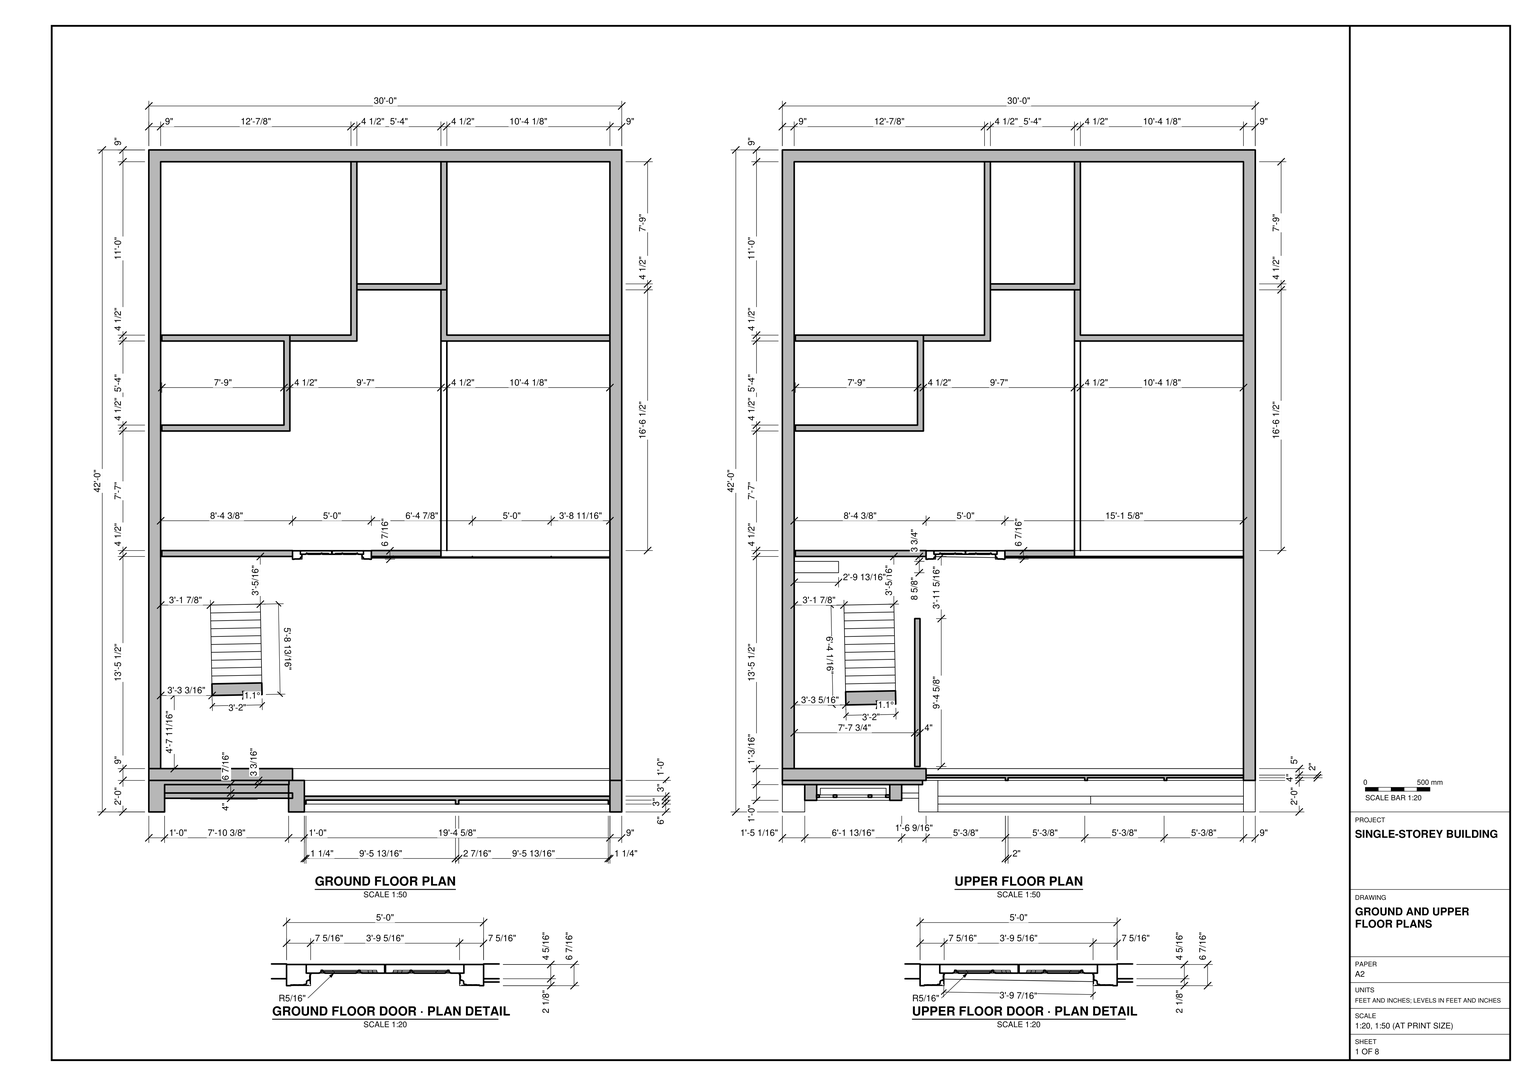
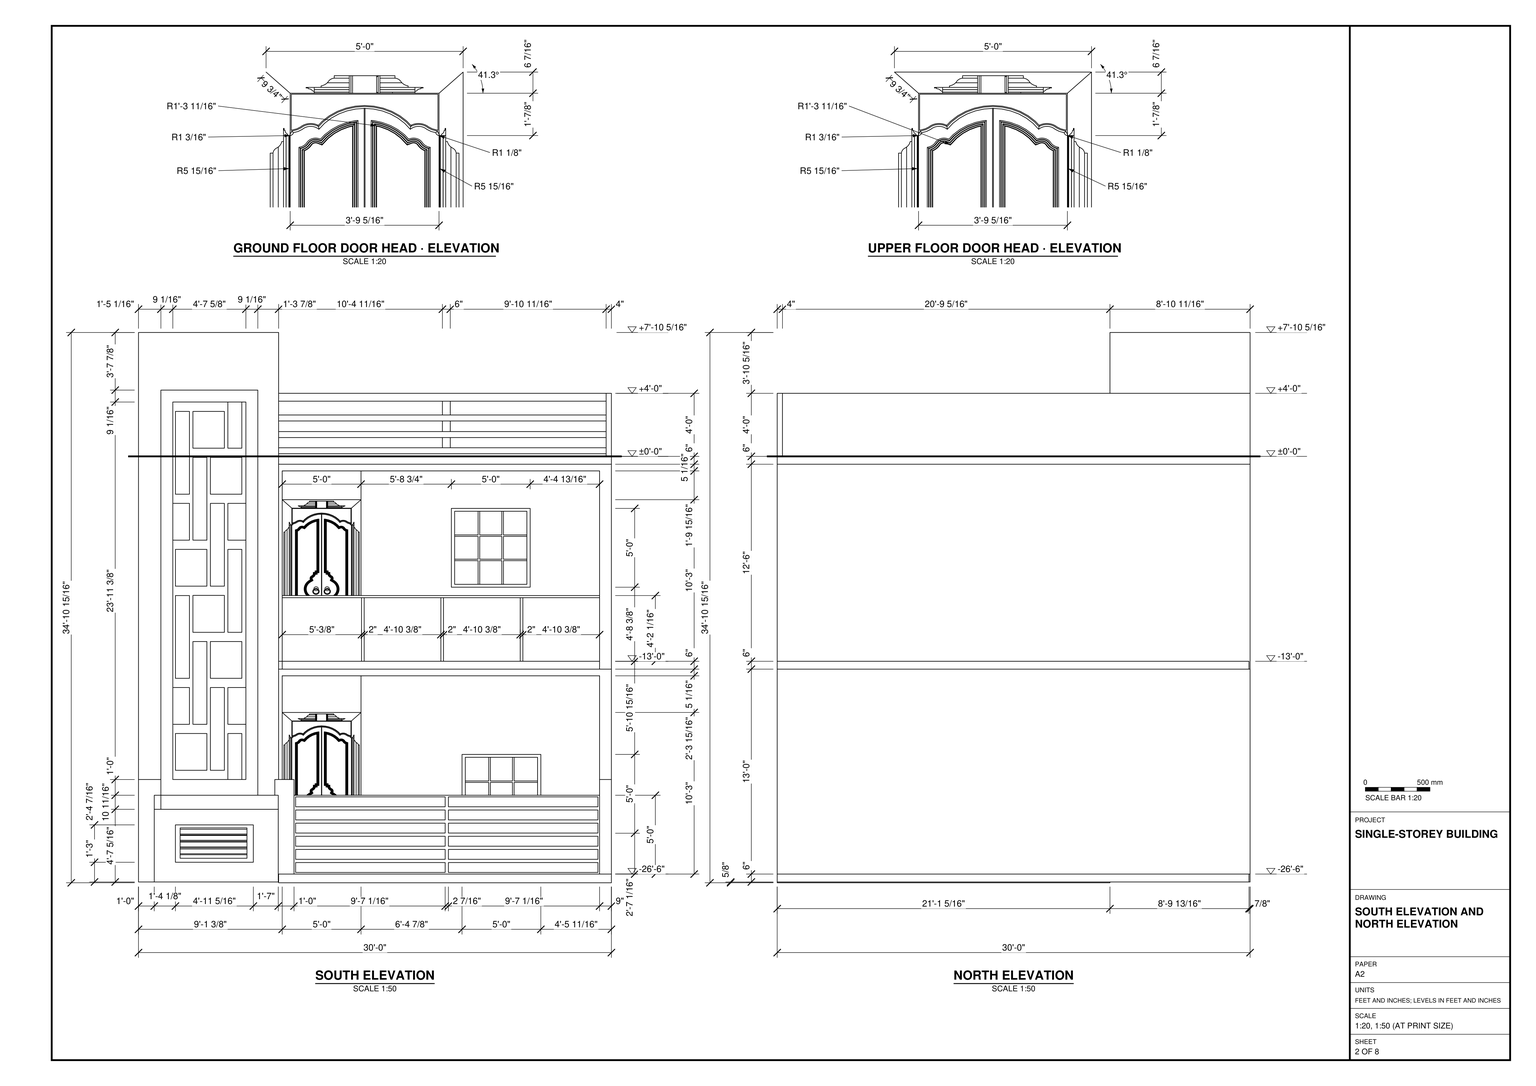
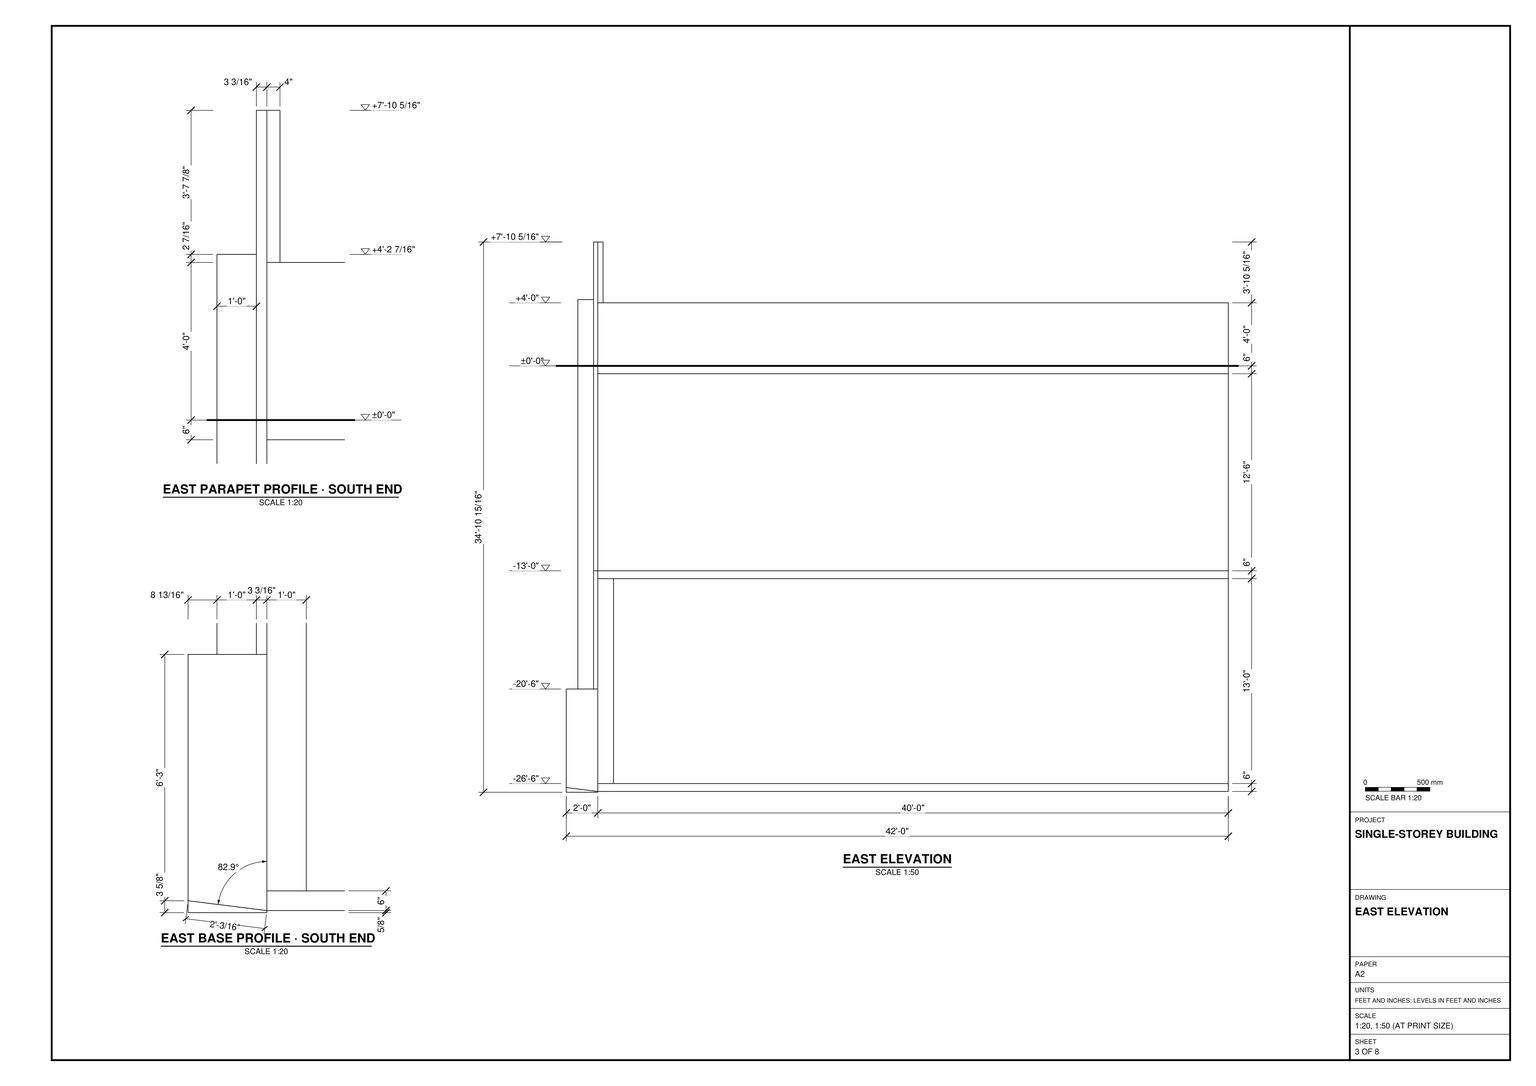
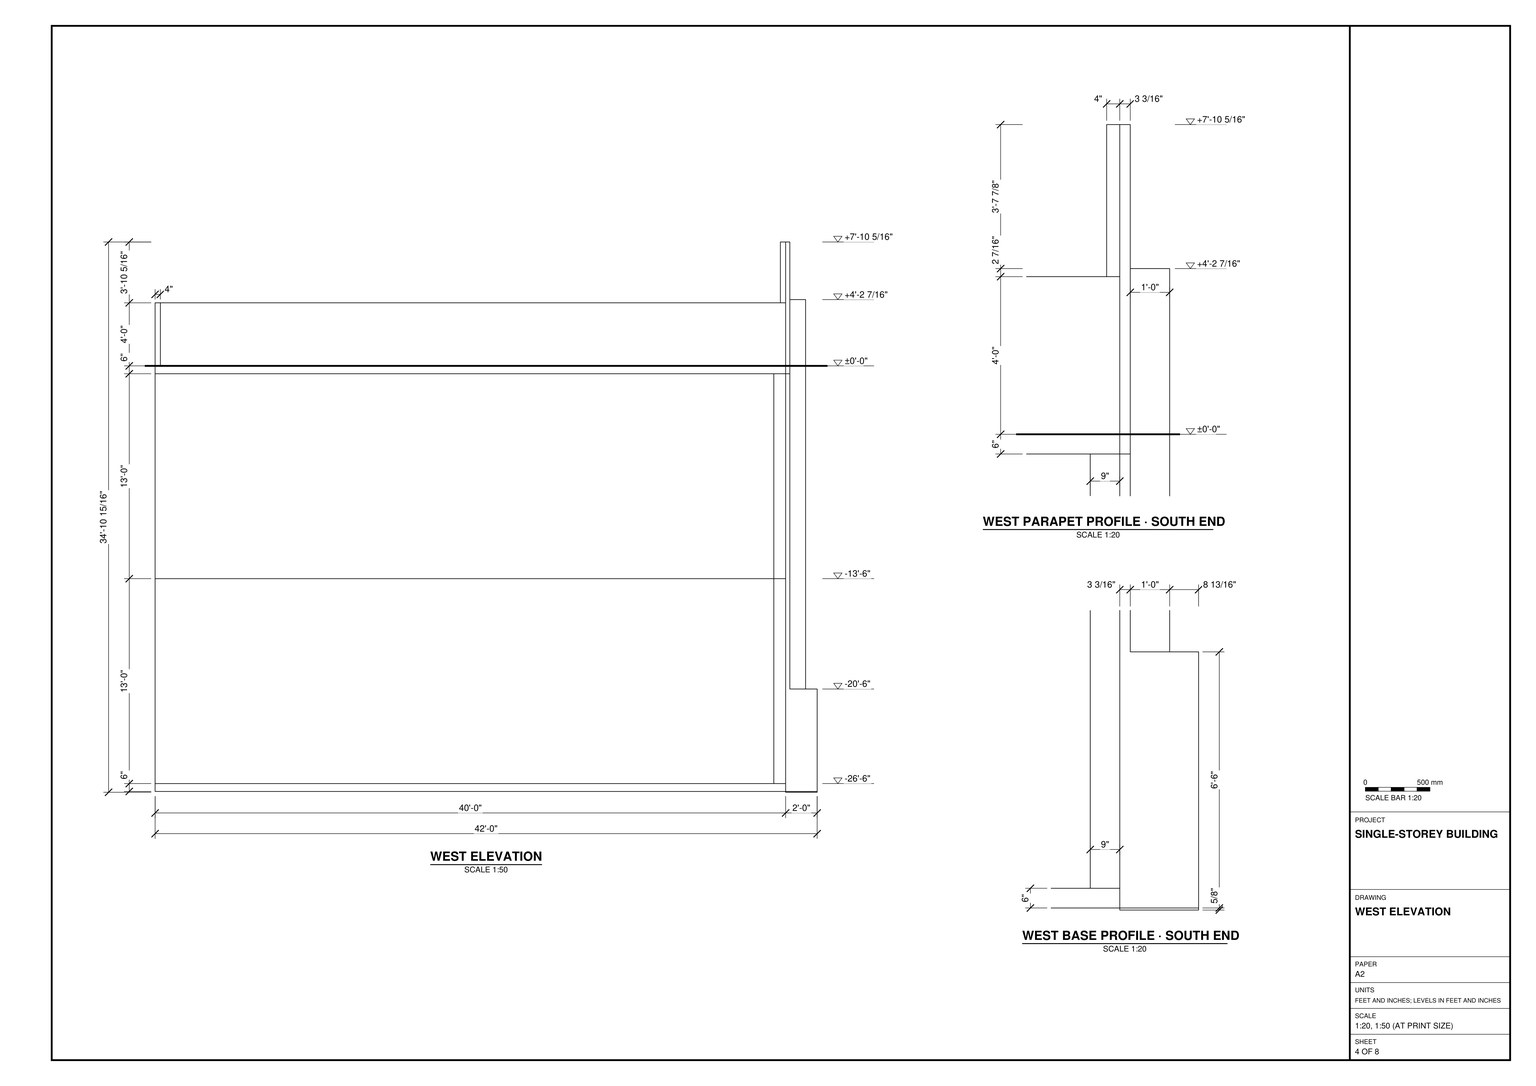
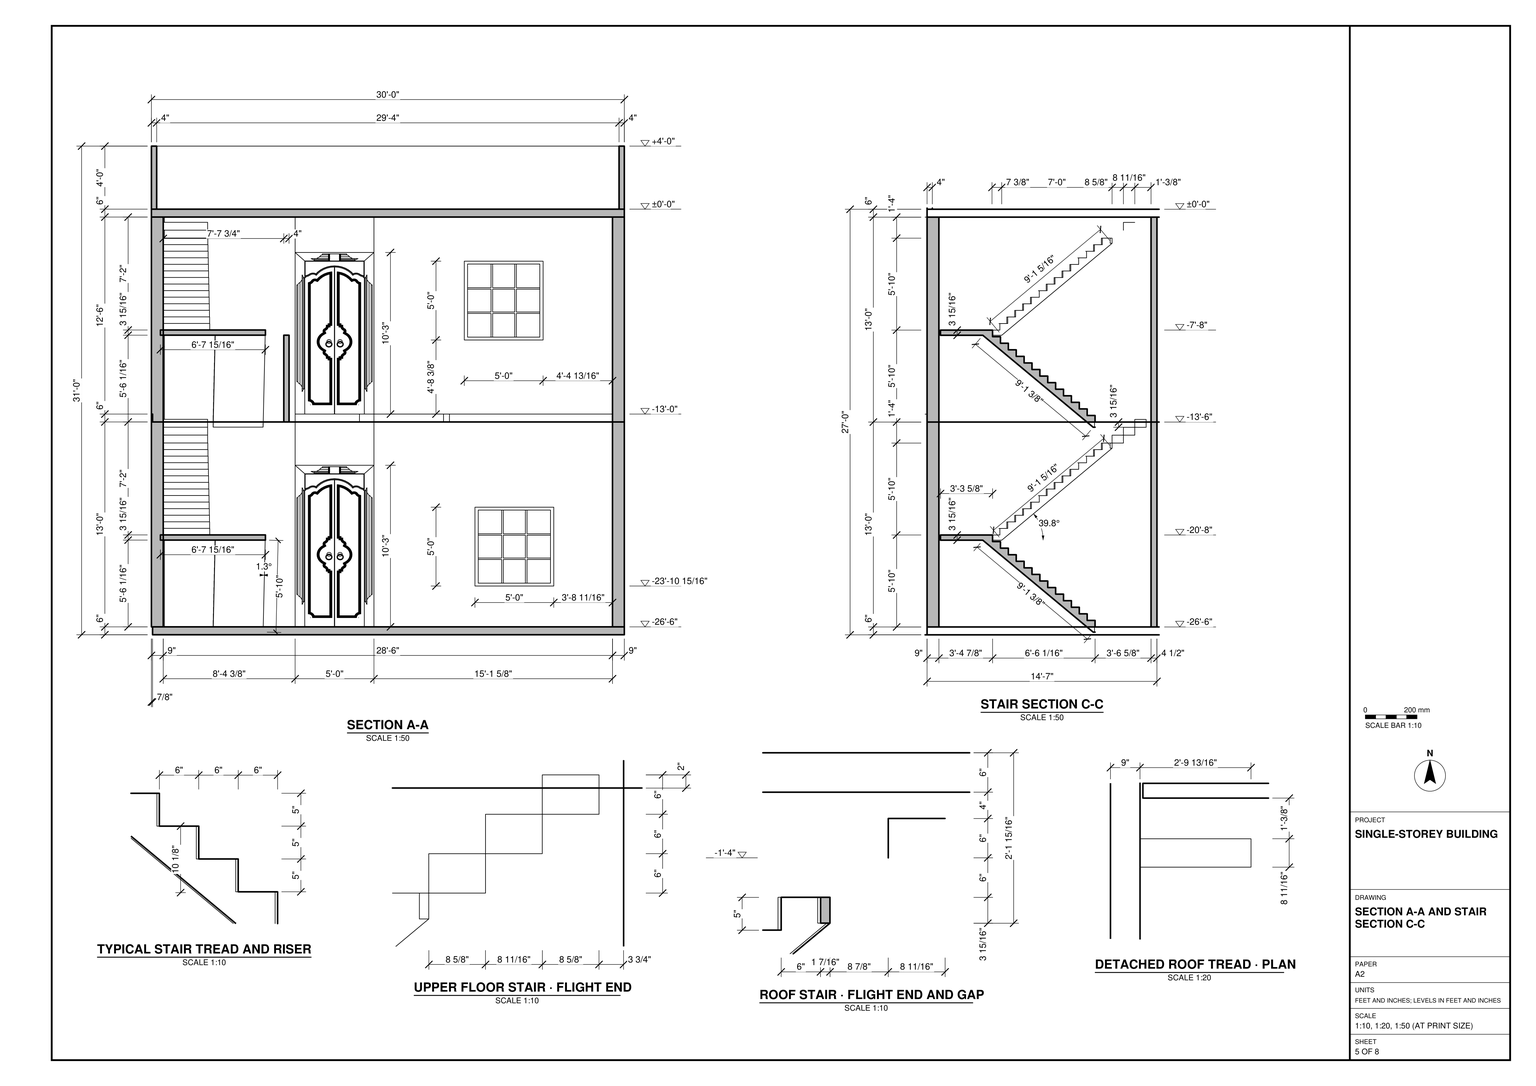
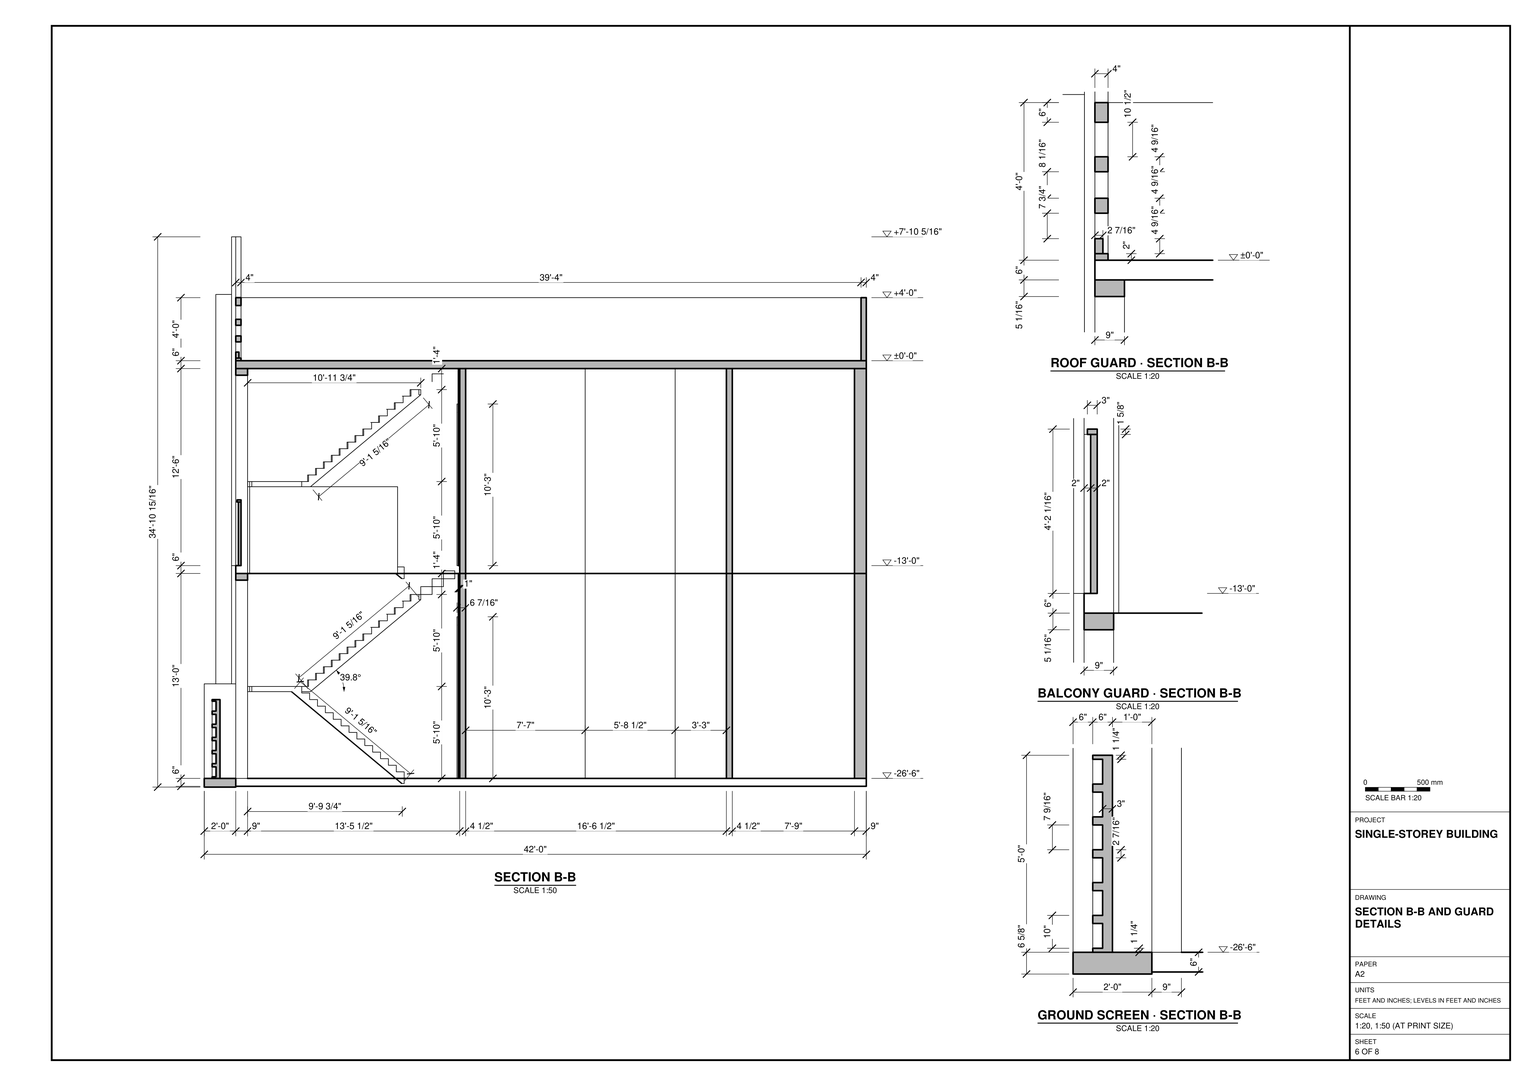
Build the ground and upper floors in SketchUp from task_files/diagram_01.pdf. Work in feet and inches. The building is 30'-0" wide across the south front, 42'-0" deep and 34'-10 15/16" high overall. Use the elevation datum marked ±0'-0" at the roof slab and place the floor slabs below it as drawn.

Lay out the 9" exterior walls and 4 1/2" interior partitions from the two plans. Keep the broad front bay, the stair on its left and the partitioned rooms at the rear. Model the slabs, stair openings, flights and landings so their positions agree between floors. Include built-in joinery and main furniture only where shown.

Use the south elevation to align the recessed doors and windows behind the ground-floor gate and upper balcony. Follow the door-head details, window subdivisions and balcony panel spacing. Model the tall framed screen at the left of the frontage, its louvred base and its projection above the roof parapet. Decor and loose items may be any suitable library components.

Keep shell elements such as walls, slabs and roof, and each furniture or joinery piece, in separate groups or components. Use components for repeated parts. Save one SketchUp model as output_files/two_storey_building_recessed_balcony_screened_frontage.skp.

# SketchUp Ruby script. Lengths in inches.
U = 1.inch
M = Sketchup.active_model
def pt(a) = Geom::Point3d.new(a.map { |v| v * U })
def face(e, loops, mat)
  f = e.add_face(loops[0].map { |a| pt(a) })
  loops[1..].each { |l| e.add_face(l.map { |a| pt(a) }).erase! }
  f.material = f.back_material = mat if mat
  f
end
# faces: each face lists its corners as indices into pts; further lists are holes
def faces(e, pts, list, mat = nil) = list.each { |f| face(e, (f[0].is_a?(Array) ? f : [f]).map { |l| l.map { |i| pts[i] } }, mat) }
# xy, xz, yz: faces in a plane at the given z, y or x. An outline is a flat list of corners, or four numbers for a rectangle; further outlines are holes
def ring(l) = l.size == 4 ? [[l[0], l[1]], [l[2], l[1]], [l[2], l[3]], [l[0], l[3]]] : l.each_slice(2).to_a
def flat(e, list, mat, &to3) = list.each { |f| face(e, (f[0].is_a?(Array) ? f : [f]).map { |l| ring(l).map { |u, v| to3.(u, v) } }, mat) }
def xy(e, z, list, mat = nil) = flat(e, list, mat) { |x, y| [x, y, z] }
def xz(e, y, list, mat = nil) = flat(e, list, mat) { |x, z| [x, y, z] }
def yz(e, x, list, mat = nil) = flat(e, list, mat) { |y, z| [x, y, z] }
def lines(e, pts, list) = list.each { |a, b| e.add_line(pt(pts[a]), pt(pts[b])) }
# prism: a flat outline (further loops are holes) pulled along v
def prism(e, loops, v, mat = nil)
  f = face(e, loops, mat); d = Geom::Vector3d.new(v.map { |x| x * U })
  f.pushpull(f.normal.samedirection?(d) ? d.length : -d.length)
end
def box(e, o, s, mat = nil) = prism(e, [[o, [o[0] + s[0], o[1], o[2]], [o[0] + s[0], o[1] + s[1], o[2]], [o[0], o[1] + s[1], o[2]]]], [0, 0, s[2]], mat)
def at(x, y, z, deg = 0) = Geom::Transformation.translation(pt([x, y, z])) * Geom::Transformation.rotation(ORIGIN, Z_AXIS, deg.degrees)
def axes(o, x, y, z) = Geom::Transformation.new([*x, 0, *y, 0, *z, 0, *pt(o).to_a, 1])
def part(name) = M.definitions.add(name)
# library, detail: a bought-in or finely detailed component or shape, given as its bounding box
def library(name, o, s) = part(name).tap { |d| box(d.entities, o, s) }
def detail(e, o, s) = box(e.add_group.entities, o, s)
def put(e, d, t, mat = nil) = e.add_instance(d, t).tap { |i| i.material = mat if mat }
def group(e, t, mat = nil) = e.add_group.tap { |g| g.transformation = t; g.material = mat if mat }.entities
root = M.entities
M.materials.add("[Color C08]").color = [102, 51, 0]
M.materials.add("[Color E02]").color = [255, 255, 153]
M.materials.add("[Color M08]").color = [30, 30, 30]
M.materials.add("[Color M09]").color = [0, 0, 0]
M.materials.add("[Formica Laminate Dark]").color = [50, 53, 60]
M.materials.add("[Translucent Glass Gray]").color = [128, 128, 128]
M.materials["[Translucent Glass Gray]"].alpha = 0.5
M.materials.add("[Translucent_Glass_Gray]").color = [128, 128, 128]
M.materials["[Translucent_Glass_Gray]"].alpha = 0.5
M.materials.add("[Wood Bamboo]").color = [177, 105, 43]
M.materials.add("[Wood Cherry Original]").color = [152, 86, 42]
M.materials.add("elevation light").color = [247, 199, 75]
c1 = library("Decorative panel door",[0,0,0],[4.33,35.43,82.68])
c2 = part("window4x4x7")
xz(c2.entities,0,[[[-24,0,24,55],[-22,2,22,53]],[[-7.72,2,-6.72,2,-6.72,18.53,6.72,18.53,6.72,2,7.72,2,7.72,18.53,22,18.53,22,19.53,7.72,19.53,7.72,35.47,22,35.47,22,36.47,7.72,36.47,7.72,53,6.72,53,6.72,36.47,-6.72,36.47,-6.72,53,-7.72,53,-7.72,36.47,-22,36.47,-22,35.47,-7.72,35.47,-7.72,19.53,-22,19.53,-22,18.53,-7.72,18.53],[-6.72,19.53,6.72,35.47]]],"[Color M08]")
xz(c2.entities,0,[[-22,2,-7.72,18.53],[-6.72,2,6.72,18.53],[7.72,2,22,18.53],[-22,19.53,-7.72,35.47],[-6.72,19.53,6.72,35.47],
  [7.72,19.53,22,35.47],[-22,36.47,-7.72,53],[-6.72,36.47,6.72,53],[7.72,36.47,22,53]],"[Translucent_Glass_Gray]")
c3 = part("Group11\#2")
xy(c3.entities,-3.9375,[[139.62,23.88,177.62,25.3]])
xy(c3.entities,0,[[139.62,17.88,177.62,23.88]])
xy(c3.entities,5,[[139.62,23.88,177.62,29.88]])
xy(c3.entities,10,[[139.62,29.88,177.62,35.88]])
xy(c3.entities,15,[[139.62,35.88,177.62,41.88]])
xy(c3.entities,20,[[139.62,41.88,177.62,47.88]])
xy(c3.entities,25,[[139.62,47.88,177.62,53.88]])
xy(c3.entities,30,[[139.62,53.88,177.62,59.88]])
xy(c3.entities,35,[[139.62,59.88,177.62,65.88]])
xy(c3.entities,40,[[139.62,65.88,177.62,71.88]])
xy(c3.entities,45,[[139.62,71.88,177.62,77.88]])
xy(c3.entities,50,[[139.62,77.88,177.62,83.88]])
xy(c3.entities,55,[[139.62,83.88,177.62,89.88]])
xy(c3.entities,60,[[139.62,89.88,177.62,95.88]])
xy(c3.entities,65,[[139.62,95.88,177.62,101.88]])
xy(c3.entities,66.0625,[[181.55,94.45,181.55,101.88,177.62,101.88,177.62,109.3,139.62,109.3,139.62,139.88,219.55,139.88,219.55,94.45],[139.62,139.88,219.55,141.53]])
xy(c3.entities,70,[[181.55,95.88,219.55,95.88,219.55,141.53,139.62,141.53,139.62,101.88,181.55,101.88]])
xy(c3.entities,75,[[181.55,89.88,219.55,95.88]])
xy(c3.entities,80,[[181.55,83.88,219.55,89.88]])
xy(c3.entities,85,[[181.55,77.88,219.55,83.88]])
xy(c3.entities,90,[[181.55,71.88,219.55,77.88]])
xy(c3.entities,95,[[181.55,65.88,219.55,71.88]])
xy(c3.entities,100,[[181.55,59.88,219.55,65.88]])
xy(c3.entities,105,[[181.55,53.88,219.55,59.88]])
xy(c3.entities,110,[[181.55,47.88,219.55,53.88]])
xy(c3.entities,115,[[181.55,41.88,219.55,47.88]])
xy(c3.entities,120,[[181.55,35.88,219.55,41.88]])
xy(c3.entities,125,[[181.55,29.88,219.55,35.88]])
xy(c3.entities,130,[[181.55,23.88,219.55,29.88]])
xy(c3.entities,135,[[181.55,17.88,219.55,23.88]])
xy(c3.entities,136.0625,[[181.55,10.45,217.12,11.88]])
xy(c3.entities,140,[[181.55,10.45,217.12,11.88],[181.55,11.88,219.55,17.88]])
xz(c3.entities,10.45,[[181.55,136.0625,217.12,140]])
xz(c3.entities,11.88,[[181.55,136.0625,217.12,140]])
xz(c3.entities,17.88,[[181.55,135,219.55,140]])
xz(c3.entities,23.88,[[139.62,0,177.62,5],[181.55,130,219.55,135]])
xz(c3.entities,29.88,[[139.62,5,177.62,10],[181.55,125,219.55,130]])
xz(c3.entities,35.88,[[139.62,10,177.62,15],[181.55,120,219.55,125]])
xz(c3.entities,41.88,[[139.62,15,177.62,20],[181.55,115,219.55,120]])
xz(c3.entities,47.88,[[139.62,20,177.62,25],[181.55,110,219.55,115]])
xz(c3.entities,53.88,[[139.62,25,177.62,30],[181.55,105,219.55,110]])
xz(c3.entities,59.88,[[139.62,30,177.62,35],[181.55,100,219.55,105]])
xz(c3.entities,65.88,[[139.62,35,177.62,40],[181.55,95,219.55,100]])
xz(c3.entities,71.88,[[139.62,40,177.62,45],[181.55,90,219.55,95]])
xz(c3.entities,77.88,[[139.62,45,177.62,50],[181.55,85,219.55,90]])
xz(c3.entities,83.88,[[139.62,50,177.62,55],[181.55,80,219.55,85]])
xz(c3.entities,89.88,[[139.62,55,177.62,60],[181.55,75,219.55,80]])
xz(c3.entities,95.88,[[139.62,60,177.62,65],[181.55,70,219.55,75]])
xz(c3.entities,101.88,[[139.62,65,177.62,70],[177.62,66.0625,181.55,70]])
xz(c3.entities,141.53,[[139.62,66.0625,219.55,70]])
yz(c3.entities,139.62,[[23.88,-3.9375,23.88,5,29.88,5,29.88,10,35.88,10,35.88,15,41.88,15,41.88,20,47.88,20,47.88,25,53.88,25,53.88,30,59.88,30,59.88,35,65.88,35,65.88,40,71.88,40,71.88,45,77.88,45,77.88,50,83.88,50,83.88,55,89.88,55,89.88,60,95.88,60,95.88,65,101.88,65,101.88,70,139.88,70,139.88,66.0625,109.3,66.0625,25.3,-3.9375],[139.88,66.0625,141.53,70]])
yz(c3.entities,177.62,[[23.88,-3.9375,25.3,-3.9375,109.3,66.0625,101.88,66.0625,101.88,65,95.88,65,95.88,60,89.88,60,89.88,55,83.88,55,83.88,50,77.88,50,77.88,45,71.88,45,71.88,40,65.88,40,65.88,35,59.88,35,59.88,30,53.88,30,53.88,25,47.88,25,47.88,20,41.88,20,41.88,15,35.88,15,35.88,10,29.88,10,29.88,5,23.88,5]])
yz(c3.entities,181.55,[[94.45,66.0625,10.45,136.0625,11.88,136.0625,11.88,140,17.88,140,17.88,135,23.88,135,23.88,130,29.88,130,29.88,125,35.88,125,35.88,120,41.88,120,41.88,115,47.88,115,47.88,110,53.88,110,53.88,105,59.88,105,59.88,100,65.88,100,65.88,95,71.88,95,71.88,90,77.88,90,77.88,85,83.88,85,83.88,80,89.88,80,89.88,75,95.88,75,95.88,70,101.88,70,101.88,66.0625],[10.45,136.0625,11.88,140]])
yz(c3.entities,217.12,[[10.45,136.0625,11.88,136.0625,11.88,140],[10.45,136.0625,11.88,140,10.45,140]])
yz(c3.entities,219.55,[[94.45,66.0625,139.88,66.0625,139.88,70,95.88,70,95.88,75,89.88,75,89.88,80,83.88,80,83.88,85,77.88,85,77.88,90,71.88,90,71.88,95,65.88,95,65.88,100,59.88,100,59.88,105,53.88,105,53.88,110,47.88,110,47.88,115,41.88,115,41.88,120,35.88,120,35.88,125,29.88,125,29.88,130,23.88,130,23.88,135,17.88,135,17.88,140,11.88,140,11.88,136.0625,10.45,136.0625],[139.88,66.0625,141.53,70]])
p = [[139.62,25.3,-3.9375],[139.62,109.3,66.0625],[177.62,109.3,66.0625],[177.62,25.3,-3.9375],[219.55,94.45,66.0625],[219.55,10.45,136.0625],
  [217.12,10.45,136.0625],[181.55,10.45,136.0625],[181.55,94.45,66.0625]]
faces(c3.entities,p,[[0,1,2,3],[4,5,6,7,8]])
c4 = part("Group11\#1")
box(c4.entities,[9,186.5,0],[99.52,4.5,156])
c5 = part("Group12\#1")
prism(c5.entities,[[[102,286.5,0],[102,350.5,0],[9,350.5,0],[9,355,0],[106.5,355,0],[106.5,282,0],[9,282,0],[9,286.5,0]]],[0,0,156])
c6 = part("Group13\#1")
prism(c6.entities,[[[106.5,355,0],[153,355,0],[153,487,0],[157.5,487,0],[157.5,350.5,0],[106.5,350.5,0]]],[0,0,156])
c7 = part("Group14\#1")
prism(c7.entities,[[[157.5,394,0],[221.5,394,0],[221.5,487,0],[226,487,0],[226,389.5,0],[157.5,389.5,0]]],[0,0,156])
c8 = part("Group15\#1")
prism(c8.entities,[[[226,389.5,0],[226,355,0],[350.125,355,0],[350.125,350.5,0],[221.5,350.5,0],[221.5,389.5,0]]],[0,0,156])
c9 = part("Group7\#1")
g1 = group(c9.entities,at(0,16,0))
xy(g1,0,[[0,0,109.4,9],[351,0,351,471,9,471,9,9,0,9,0,480,360,480,360,0],[9,9,351,471]])
xy(g1,150.9375,[[109.4,0,351,9]])
xy(g1,156,[[0,0,360,0,360,480,0,480,0,9,9,9,9,471,351,471,351,9,0,9]])
xz(g1,0,[[0,0,109.4,0,109.4,150.9375,351,150.9375,351,0,360,0,360,156,0,156]],"[Color C08]")
xz(g1,9,[[0,0,0,156,351,156,351,150.9375,109.4,150.9375,109.4,0],[0,0,9,156]])
xz(g1,471,[[9,0,351,156]])
xz(g1,480,[[0,0,360,156]])
yz(g1,0,[[0,0,9,156],[9,0,480,156]])
yz(g1,9,[[9,0,471,156]])
yz(g1,109.4,[[0,0,9,150.9375]])
yz(g1,351,[[0,0,9,1.6875],[9,0,471,156]])
yz(g1,351,[[0,1.6875,9,150.9375]],"[Color C08]")
yz(g1,360,[[12,0,480,156]])
yz(g1,360,[[0,0,12,156]],"[Color C08]")
c10 = part("Group18\#1")
box(c10.entities,[168.52,182,0],[52.98,4.5,156])
c11 = part("Group16\#2")
xy(c11.entities,0,[[221.5,191,226,350.5]])
xy(c11.entities,156,[[221.5,191,226,350.5]])
xz(c11.entities,350.5,[[221.5,0,226,156]])
yz(c11.entities,221.5,[[191,0,350.5,156]])
yz(c11.entities,226,[[191,0,350.5,156]])
# 3 loose lines left out
c12 = part("Group16\#1")
xy(c12.entities,0,[[221.5,191,226,350.5]])
xy(c12.entities,156,[[221.5,191,226,350.5]])
xz(c12.entities,350.5,[[221.5,0,226,156]])
yz(c12.entities,221.5,[[191,0,350.5,156]])
yz(c12.entities,226,[[191,0,350.5,156]])
# 3 loose lines left out
c13 = part("Group18\#2")
box(c13.entities,[168.52,182,0],[52.98,4.5,156])
c14 = part("Group7\#2")
g2 = group(c14.entities,at(0,16,0))
xy(g2,0,[[0,0,109.4,9],[351,0,351,471,9,471,9,9,0,9,0,480,360,480,360,0],[9,9,351,471]])
xy(g2,150.9375,[[109.4,0,351,9]])
xy(g2,156,[[0,0,360,0,360,480,0,480,0,9,9,9,9,471,351,471,351,9,0,9]])
xz(g2,0,[[0,0,109.4,0,109.4,150.9375,351,150.9375,351,0,360,0,360,156,0,156]])
xz(g2,9,[[0,0,0,156,351,156,351,150.9375,109.4,150.9375,109.4,0],[0,0,9,156]])
xz(g2,471,[[9,0,351,156]])
xz(g2,480,[[0,0,360,156]])
yz(g2,0,[[0,0,9,156],[9,0,480,156]])
yz(g2,9,[[9,0,471,156]])
yz(g2,109.4,[[0,0,9,150.9375]])
yz(g2,351,[[0,0,9,150.9375],[9,0,471,156]])
yz(g2,360,[[0,0,480,156]])
xy(root,-6.625,[[106.6875,0,360,24]])
xy(root,-6,[[0,0,0,24,106.6875,24,106.6875,20.8125,12,20.8125,12,0],[12,10.41,106.4,14.41],[0.875,24,360,504]])
xy(root,0,[[106.4,0,106.6875,10.41],[118.4,0,351,6],[118.4,6,351,12],[106.4,10.41,106.6875,14.41],[106.6875,10.41,109.4,14.41],
  [118.4,12,351,24],[106.4,14.41,106.6875,20.8125]])
xy(root,1.23,[[119.625,6,233.47,9],[235.93,6,349.77,9]])
xy(root,8.77,[[119.625,6,233.47,9],[235.93,6,349.77,9]],"[Color M09]")
xy(root,11.23,[[119.625,6,233.47,9],[235.93,6,349.77,9]],"[Color M09]")
xy(root,12.02,[[31.7,10.41,82.58,14.41]])
xy(root,18.77,[[119.625,6,233.47,9],[235.93,6,349.77,9]],"[Color M09]")
xy(root,21.23,[[119.625,6,233.47,9],[235.93,6,349.77,9]],"[Color M09]")
xy(root,28.77,[[119.625,6,233.47,9],[235.93,6,349.77,9]],"[Color M09]")
xy(root,31.09,[[246.29,193.5,306.29,194.5]])
xy(root,31.23,[[119.625,6,233.47,9],[235.93,6,349.77,9]],"[Color M09]")
xy(root,35.15,[[31.7,10.41,82.58,14.41]],"[Color M09]")
xy(root,38.77,[[119.625,6,233.47,9],[235.93,6,349.77,9]],"[Color M09]")
xy(root,41.23,[[119.625,6,233.47,9],[235.93,6,349.77,9]],"[Color M09]")
xy(root,48.77,[[119.625,6,233.47,9],[235.93,6,349.77,9]],"[Color M09]")
xy(root,49.3125,[[12,10.41,17.04,14.41],[17.04,10.41,109.4,14.41]])
xy(root,51.23,[[119.625,6,233.47,9],[235.93,6,349.77,9]],"[Color M09]")
xy(root,58.77,[[119.625,6,233.47,9],[235.93,6,349.77,9]],"[Color M09]")
xy(root,60,[[12,0,17.04,10.41],[103.79,0,106.4,20.8125],[118.4,6,234.7,12],[234.7,6,351,12],[17.04,8.8125,26.125,20.8125],
  [26.125,8.8125,81.75,20.8125],[81.75,8.8125,90.83,20.8125],[12,14.41,17.04,20.8125]])
xy(root,72,[[0,0,17.04,20.8125],[103.79,0,118.4,0,118.4,24,106.6875,24,106.6875,20.8125,103.79,20.8125],[351,0,360,24],[[26.125,8.8125,81.75,20.8125],[28.9,11.59,78.97,18.04]]])
xy(root,72,[[28.9,11.59,78.97,18.04]],"elevation light")
xy(root,91.09,[[246.29,193.5,306.29,194.5]])
xy(root,140,[[8.97,164.83,42.8,173.47]])
xy(root,146,[[8.97,164.83,42.8,173.47],[8.97,173.47,42.8,182.11]])
xy(root,152,[[8.97,173.47,42.8,182.11],[8.97,182.11,42.8,190.76]])
xy(root,156,[[[0.875,24,360,504],[100.78,34.57,104.78,147.19]]])
xy(root,158,[[8.97,182.11,42.8,190.76]])
xy(root,162,[[109.4,24,169.8,26],[169.8,24,171.8,24,171.8,26,230.2,26,230.2,24,232.2,24,232.2,26,290.6,26,290.6,24,292.6,24,292.6,26,351,26,351,28,109.4,28,109.4,26,169.8,26],[171.8,24,230.2,26],[232.2,24,290.6,26],[292.6,24,351,26],
  [169.4,193.5,351,194.5]])
xy(root,210.42,[[109.4,25,169.8,26],[171.8,25,230.2,26],[232.2,25,290.6,26],[292.6,25,351,26]])
xy(root,210.42,[[169.8,24,171.8,25],[230.2,24,232.2,25],[290.6,24,292.6,25],[169.8,25,171.8,26],[230.2,25,232.2,26],
  [290.6,25,292.6,26],[109.4,26,351,28]],"[Formica Laminate Dark]")
xy(root,212.04,[[109.4,25,351,28]],"[Formica Laminate Dark]")
xy(root,218.4,[[238.17,193.5,298.17,194.5]])
xy(root,222.0625,[[100.78,34.57,104.78,147.19]])
xy(root,278.4,[[238.17,193.5,298.17,194.5]])
xy(root,308,[[8.97,173.47,42.8,182.11]])
xy(root,312,[[0,24,360,504],[169.4,193.5,351,194.5]])
xy(root,318,[[0,24,4,500],[4,24,106.6875,28],[106.6875,24,356,28],[356,24,360,504],[4,28,356,500],
  [0,500,356,504]])
xy(root,320,[[106.6875,24,356,26.4375],[106.6875,26.4375,356,28]])
xy(root,324.5625,[[106.6875,24,231.34,26.4375],[231.34,24,237.34,26.4375],[237.34,24,356,26.4375],[231.34,26.4375,237.34,28]])
xy(root,332.3125,[[106.6875,24,231.34,28],[231.34,24,237.34,28],[237.34,24,356,28]])
xy(root,336.875,[[106.6875,24,231.34,28],[231.34,24,237.34,28],[237.34,24,356,28]])
xy(root,344.9375,[[106.6875,24,231.34,28],[231.34,24,237.34,28],[237.34,24,356,28]])
xy(root,349.5,[[106.6875,24,231.34,28],[231.34,24,237.34,28],[237.34,24,356,28]])
xy(root,359.375,[[[26.125,8.8125,81.75,20.8125],[28.9,11.59,78.97,18.04]]])
xy(root,359.375,[[28.9,11.59,78.97,18.04]],"elevation light")
xy(root,360,[[106.6875,24,231.34,28],[231.34,24,237.34,28],[237.34,24,356,28]])
xy(root,366,[[0,24,4,28],[106.6875,24,356,28],[356,24,360,504],[0,28,4,500],[0,500,356,504]])
xy(root,368.46,[[17.04,8.8125,90.83,20.8125]])
xy(root,412.3125,[[0,20.8125,106.6875,24],[0,24,106.6875,28]])
xz(root,0,[[106.6875,-6.625,360,0],[0,-6,12,-6,12,60,17.04,60,17.04,72,0,72],[106.4,0,118.4,0,118.4,72,103.79,72,103.79,60,106.4,60],[351,0,360,72]])
xz(root,6,[[[118.4,0,351,60],[235.93,51.23,349.77,58.77],[235.93,41.23,349.77,48.77],[235.93,31.23,349.77,38.77],[235.93,21.23,349.77,28.77],[235.93,11.23,349.77,18.77],[235.93,1.23,349.77,8.77],[119.625,21.23,233.47,28.77],[119.625,1.23,233.47,8.77],[119.625,11.23,233.47,18.77],[119.625,31.23,233.47,38.77],[119.625,41.23,233.47,48.77],[119.625,51.23,233.47,58.77]]],"[Color M09]")
xz(root,8.8125,[[[17.04,60,90.83,368.46],[26.125,72,81.75,359.375]]])
xz(root,9,[[119.625,1.23,233.47,8.77],[235.93,1.23,349.77,8.77],[119.625,11.23,233.47,18.77],[235.93,11.23,349.77,18.77],[119.625,21.23,233.47,28.77],
  [235.93,21.23,349.77,28.77],[119.625,31.23,233.47,38.77],[235.93,31.23,349.77,38.77],[119.625,41.23,233.47,48.77],[235.93,41.23,349.77,48.77],
  [119.625,51.23,233.47,58.77],[235.93,51.23,349.77,58.77]],"[Wood Bamboo]")
xz(root,10.41,[[[12,-6,106.4,-6,106.4,0,109.4,0,109.4,49.3125,12,49.3125],[28.1,9.01,87.42,37.44]],[12,49.3125,17.04,60]])
xz(root,10.41,[[[28.1,9.01,87.42,37.44],[31.7,12.02,82.58,35.15]]],"[Color M09]")
xz(root,12,[[118.4,0,351,60]])
xz(root,14.41,[[[12,-6,12,49.3125,109.4,49.3125,109.4,0,106.4,0,106.4,-6],[31.7,12.02,82.58,35.15]],[31.7,12.02,82.58,19.1],[31.7,19.1,82.58,23.59],[31.7,23.59,82.58,29.37],[31.7,29.37,82.58,34.1],
  [31.7,34.1,82.58,35.15],[12,49.3125,17.04,60]])
xz(root,20.8125,[[12,-6,106.4,60],[106.4,-6,106.6875,0],[106.4,0,106.6875,60],[17.04,60,26.125,60,26.125,359.375,81.75,359.375,81.75,60,90.83,60,90.83,368.46,17.04,368.46],[103.79,60,106.6875,72],
  [26.125,72,81.75,359.375]])
xz(root,20.8125,[[90.83,60,103.79,60,103.79,72,106.6875,72,106.6875,412.3125,0,412.3125,0,72,17.04,72,17.04,368.46,90.83,368.46]],"[Color E02]")
xz(root,24,[[106.6875,-6.625,360,-6],[0,-6,0.875,0],[0.875,-6,106.6875,0],[106.6875,-6,360,0],[106.6875,0,118.4,72],
  [351,0,360,72],[0.875,156,106.6875,162],[0,312,106.6875,318],[106.6875,312,360,318],[0,318,4,366],
  [4,318,106.6875,318,106.6875,412.3125,0,412.3125,0,366,4,366],[106.6875,318,356,320],[356,318,360,366],[106.6875,320,356,324.5625],[231.34,324.5625,237.34,332.3125],
  [106.6875,332.3125,356,336.875],[231.34,336.875,237.34,344.9375],[106.6875,344.9375,356,349.5],[231.34,349.5,237.34,360],[106.6875,360,356,366]])
xz(root,24,[[106.6875,156,351,162],[169.8,162,171.8,210.42],[230.2,162,232.2,210.42],[290.6,162,292.6,210.42]],"[Formica Laminate Dark]")
xz(root,25,[[109.4,210.42,351,212.04]],"[Formica Laminate Dark]")
xz(root,26,[[109.4,162,169.8,210.42],[171.8,162,230.2,210.42],[232.2,162,290.6,210.42],[292.6,162,351,210.42]],"[Translucent Glass Gray]")
xz(root,26.4375,[[106.6875,320,356,324.5625]])
xz(root,28,[[109.4,210.42,351,212.04],[4,318,4,366,0,366,0,412.3125,106.6875,412.3125,106.6875,318],[106.6875,318,356,320],[231.34,324.5625,237.34,332.3125],[106.6875,332.3125,356,336.875],
  [231.34,336.875,237.34,344.9375],[106.6875,344.9375,356,349.5],[231.34,349.5,237.34,360],[106.6875,360,356,366]])
xz(root,28,[[109.4,162,351,210.42]],"[Translucent Glass Gray]")
xz(root,34.57,[[100.78,156,104.78,222.0625]])
xz(root,147.19,[[100.78,156,104.78,222.0625]])
xz(root,164.83,[[8.97,140,42.8,146]])
xz(root,173.47,[[8.97,140,42.8,146],[8.97,146,42.8,152],[8.97,302,42.8,308]])
xz(root,182.11,[[8.97,146,42.8,152],[8.97,152,42.8,158]])
xz(root,190.76,[[8.97,152,42.8,158]])
xz(root,193.5,[[[169.4,0,351,156],[246.29,31.09,306.29,91.09]],[[169.4,162,351,312],[238.17,218.4,298.17,278.4]]],"[Color E02]")
xz(root,194.5,[[[169.4,162,351,312],[238.17,218.4,298.17,278.4]]])
xz(root,500,[[0,318,4,366],[4,318,356,366]])
xz(root,504,[[0.875,-6,360,0],[0.875,156,360,162],[0,312,360,318],[0,318,356,366],[356,318,360,366]])
yz(root,0,[[0,-6,0,72,20.8125,72,20.8125,312,24,312,24,-6],[20.8125,312,24,412.3125],[24,312,504,318],[24,318,500,366],[500,318,504,366],
  [24,366,28,412.3125]])
yz(root,0.875,[[24,-6,504,0],[24,156,504,162]])
yz(root,4,[[24,318,28,366],[28,318,500,366]])
yz(root,8.97,[[164.83,140,173.47,146],[173.47,146,182.11,152],[182.11,152,190.76,158]])
yz(root,12,[[0,-6,10.41,60],[10.41,-6,14.41,49.3125],[14.41,-6,20.8125,60]])
yz(root,17.04,[[10.41,49.3125,14.41,60],[0,60,8.8125,72],[8.8125,60,20.8125,72],[8.8125,72,20.8125,368.46]])
yz(root,26.125,[[[8.8125,72,20.8125,359.375],[11.59,74.78,18.04,356.6]]])
yz(root,26.125,[[11.59,74.78,18.04,356.6]],"elevation light")
yz(root,31.7,[[11.08,14.73,14.41,17.75,14.41,19.1,11.08,16.08,10.41,15.47],[10.41,19.96,9.73,20.7,10.41,21.3125],[10.41,19.96,14.41,23.59,13.73,24.33,10.41,21.3125],[11.08,25,14.41,28.02,14.41,29.37,11.08,26.35,10.41,25.74],[11.08,29.73,14.41,32.75,14.41,34.1,11.08,31.08,10.41,30.47]])
yz(root,31.7,[[10.41,12.02,14.41,12.02,14.41,17.75,11.08,14.73,10.41,15.47,11.08,16.08,14.41,19.1,14.41,23.59,10.41,19.96],[10.41,21.3125,13.73,24.33,14.41,23.59,14.41,28.02,11.08,25,10.41,25.74],[10.41,25.74,11.08,26.35,14.41,29.37,14.41,32.75,11.08,29.73,10.41,30.47,11.08,31.08,14.41,34.1,14.41,35.15,10.41,35.15]],"[Color M09]")
yz(root,42.8,[[164.83,140,173.47,146],[173.47,146,182.11,152],[182.11,152,190.76,158]])
yz(root,81.75,[[[8.8125,72,20.8125,359.375],[11.59,74.78,18.04,356.6]]])
yz(root,81.75,[[11.59,74.78,18.04,356.6]],"elevation light")
yz(root,82.58,[[11.08,14.73,10.41,15.47,11.08,16.08,14.41,19.1,14.41,17.75],[10.41,19.96,10.41,21.3125,9.73,20.7],[10.41,19.96,10.41,21.3125,13.73,24.33,14.41,23.59],[11.08,25,10.41,25.74,11.08,26.35,14.41,29.37,14.41,28.02],[11.08,29.73,10.41,30.47,11.08,31.08,14.41,34.1,14.41,32.75]])
yz(root,82.58,[[10.41,12.02,10.41,15.47,11.08,14.73,14.41,17.75,14.41,12.02],[10.41,15.47,10.41,19.96,14.41,23.59,14.41,19.1,11.08,16.08],[10.41,21.3125,10.41,35.15,14.41,35.15,14.41,34.1,11.08,31.08,10.41,30.47,11.08,29.73,14.41,32.75,14.41,29.37,11.08,26.35,10.41,25.74,11.08,25,14.41,28.02,14.41,23.59,13.73,24.33]],"[Color M09]")
yz(root,90.83,[[8.8125,60,20.8125,368.46]])
yz(root,100.78,[[34.57,156,147.19,222.0625]])
yz(root,103.79,[[0,60,20.8125,72]])
yz(root,104.78,[[34.57,156,147.19,222.0625]])
yz(root,106.4,[[10.41,-6,14.41,0],[0,0,20.8125,60]])
yz(root,106.6875,[[0,-6.625,0,0,20.8125,0,20.8125,-6,24,-6,24,-6.625],[20.8125,-6,24,72],[20.8125,72,24,162],[20.8125,162,24,412.3125],[24,318,28,320],
  [24,320,26.4375,324.5625],[26.4375,320,28,320,28,332.3125,24,332.3125,24,324.5625,26.4375,324.5625],[24,332.3125,28,336.875],[24,336.875,28,344.9375],[24,344.9375,28,349.5],
  [24,349.5,28,360],[24,360,28,366],[24,366,28,412.3125]])
yz(root,109.4,[[10.41,0,14.41,49.3125],[26,162,28,210.42],[25,210.42,28,212.04]])
yz(root,118.4,[[0,0,6,0,6,60,12,60,12,0,24,0,24,72,0,72],[6,0,12,60]])
yz(root,119.625,[[6,1.23,9,8.77],[6,11.23,9,18.77],[6,21.23,9,28.77],[6,31.23,9,38.77],[6,41.23,9,48.77],
  [6,51.23,9,58.77]])
yz(root,169.4,[[193.5,0,194.5,122.59],[193.5,162,194.5,312]])
yz(root,169.8,[[24,162,26,210.42]])
yz(root,171.8,[[24,162,26,210.42]])
yz(root,230.2,[[24,162,26,210.42]])
yz(root,231.34,[[24,324.5625,28,332.3125],[24,336.875,28,344.9375],[24,349.5,28,360]])
yz(root,232.2,[[24,162,26,210.42]])
yz(root,233.47,[[6,1.23,9,8.77],[6,11.23,9,18.77],[6,21.23,9,28.77],[6,31.23,9,38.77],[6,41.23,9,48.77],
  [6,51.23,9,58.77]],"[Color M09]")
yz(root,235.93,[[6,1.23,9,8.77],[6,11.23,9,18.77],[6,21.23,9,28.77],[6,31.23,9,38.77],[6,41.23,9,48.77],
  [6,51.23,9,58.77]],"[Color M09]")
yz(root,237.34,[[24,324.5625,28,332.3125],[24,336.875,28,344.9375],[24,349.5,28,360]])
yz(root,238.17,[[193.5,218.4,194.5,278.4]])
yz(root,246.29,[[193.5,31.09,194.5,91.09]])
yz(root,290.6,[[24,162,26,210.42]])
yz(root,292.6,[[24,162,26,210.42]])
yz(root,298.17,[[193.5,218.4,194.5,278.4]])
yz(root,306.29,[[193.5,31.09,194.5,91.09]])
yz(root,349.77,[[6,1.23,9,8.77],[6,11.23,9,18.77],[6,21.23,9,28.77],[6,31.23,9,38.77],[6,41.23,9,48.77],
  [6,51.23,9,58.77]])
yz(root,351,[[0,0,24,72],[26,162,28,210.42],[193.5,162,194.5,312],[25,210.42,28,212.04]])
yz(root,356,[[24,318,28,320],[28,318,28,349.5,24,349.5,24,360,28,360,28,366,500,366,500,318],[500,318,504,366],[24,320,26.4375,324.5625],[26.4375,320,26.4375,324.5625,24,324.5625,24,332.3125,28,332.3125,28,320],
  [24,332.3125,28,336.875],[24,336.875,28,344.9375],[24,344.9375,28,349.5],[24,360,28,366]])
yz(root,360,[[0,-6.625,24,-6.625,24,-6,0,-3],[24,-6,24,72,0,72,0,-3],[24,-6,504,0],[24,156,504,162],[24,312,504,318],
  [24,318,504,366]])
# 11 loose lines left out
p = [[31.7,11.08,14.73],[82.58,11.08,14.73],[82.58,10.41,15.47],[31.7,10.41,15.47],[31.7,14.41,17.75],[31.7,15.08,18.36],
  [82.58,15.08,18.36],[82.58,14.41,17.75],[31.7,14.41,19.1],[31.7,11.08,16.08],[82.58,11.08,16.08],[82.58,14.41,19.1],
  [31.7,10.41,19.96],[82.58,10.41,19.96],[82.58,9.73,20.7],[31.7,9.73,20.7],[31.7,14.41,23.59],[82.58,14.41,23.59],
  [31.7,13.73,24.33],[31.7,10.41,21.3125],[82.58,10.41,21.3125],[82.58,13.73,24.33],[31.7,11.08,25],[82.58,11.08,25],
  [82.58,10.41,25.74],[31.7,10.41,25.74],[31.7,14.41,28.02],[31.7,15.08,28.63],[82.58,15.08,28.63],[82.58,14.41,28.02],
  [31.7,14.41,29.37],[31.7,11.08,26.35],[82.58,11.08,26.35],[82.58,14.41,29.37],[31.7,11.08,29.73],[82.58,11.08,29.73],
  [82.58,10.41,30.47],[31.7,10.41,30.47],[31.7,14.41,32.75],[31.7,15.08,33.36],[82.58,15.08,33.36],[82.58,14.41,32.75],
  [31.7,14.41,34.1],[31.7,11.08,31.08],[82.58,11.08,31.08],[82.58,14.41,34.1],[109.4,194.5,122.59],[169.4,193.5,122.59],
  [169.4,193.5,156],[109.4,194.5,156],[169.4,193.5,312],[109.4,194.5,312],[109.4,194.5,285.02],[169.4,193.5,285.02]]
faces(root,p,[[0,1,2,3],[8,9,3,2,10,11],[12,13,14,15],[18,19,15,14,20,21],[22,23,24,25],[30,31,25,24,32,33],[34,35,36,37],[42,43,37,36,44,45]],"[Color M09]")
faces(root,p,[[4,5,6,7,1,0],[12,16,17,13],[17,16,18,21],[26,27,28,29,23,22],[38,39,40,41,35,34],[46,47,48,49]])
faces(root,p,[[50,51,52,53]],"[Color E02]")
put(root,c1,axes([109.4,198.83,0],[0,-1.488,0],[1.69333,0,0],[0,0,1.488]))
put(root,c1,axes([109.4,198.83,162],[0,-1.488,0],[1.69333,0,0],[0,0,1.488]))
put(root,c2,axes([268.17,193.5,218.4],[1.25,0,0],[0,1,0],[0,0,1.09091]))
put(root,c2,axes([276.29,193.5,31.09],[1.25,0,0],[0,1,0],[0,0,1.09091]))
put(root,c3,at(224.12,178.72,0,-178.913))
put(root,c4,at(0.875,8,0))
put(root,c5,at(0.875,8,0))
put(root,c6,at(0.875,8,0))
put(root,c7,at(0.875,8,0))
put(root,c8,at(0.875,8,0))
put(root,c3,at(224.12,178.72,156,-178.913))
put(root,c9,at(0,8,0))
put(root,c5,at(0.875,8,156))
put(root,c6,at(0.875,8,156))
put(root,c8,at(0.875,8,156))
put(root,c7,at(0.875,8,156))
put(root,c4,at(0.875,8,156))
put(root,c10,at(0.875,12.5,156))
put(root,c11,at(0.875,8,156))
put(root,c12,at(0.875,8,0))
put(root,c13,at(0.875,12.5,0))
g3 = group(root,at(25.83,15.48,270.17))
xy(g3,-198.17,[[0,-4.36,42.2,-2.53],[52.84,-4.36,55.92,-2.53]])
xy(g3,-191.17,[[2.3,-4.36,26.24,-2.53],[28.9,-4.36,39.54,-2.53]])
xy(g3,-163.16,[[2.3,-4.36,26.24,-2.53],[42.2,-4.36,52.84,-2.53]])
xy(g3,-156.16,[[0.17,-4.36,12.94,-2.53],[15.6,-4.36,26.24,-2.53],[42.2,-4.36,55.92,-2.53]])
xy(g3,-128.15,[[0.17,-4.36,12.94,-2.53],[28.9,-4.36,39.54,-2.53],[42.2,-4.36,55.92,-2.53]])
xy(g3,-121.15,[[2.3,-4.36,12.94,-2.53],[28.9,-4.36,52.84,-2.53]])
xy(g3,-93.14,[[15.6,-4.36,26.24,-2.53],[28.9,-4.36,52.84,-2.53]])
xy(g3,-86.14,[[15.6,-4.36,39.54,-2.53],[42.2,-4.36,52.84,-2.53]])
xy(g3,-58.125,[[2.3,-4.36,12.94,-2.53]])
xy(g3,-57.99,[[15.6,-4.36,39.54,-2.53]])
xy(g3,-50.98,[[2.3,-4.36,26.24,-2.53],[28.9,-4.36,39.54,-2.53]])
xy(g3,-22.97,[[2.3,-4.36,26.24,-2.53],[42.2,-4.36,52.84,-2.53]])
xy(g3,-15.97,[[0.17,-4.36,12.94,-2.53],[15.6,-4.36,26.24,-2.53],[42.2,-4.36,55.92,-2.53]])
xy(g3,12.04,[[0.17,-4.36,12.94,-2.53],[28.9,-4.36,39.54,-2.53],[42.2,-4.36,55.92,-2.53]])
xy(g3,19.04,[[2.3,-4.36,12.94,-2.53],[28.9,-4.36,52.84,-2.53]])
xy(g3,47.05,[[15.6,-4.36,26.24,-2.53],[28.9,-4.36,52.84,-2.53]])
xy(g3,54.05,[[15.6,-4.36,39.54,-2.53],[42.2,-4.36,52.84,-2.53]])
xy(g3,82.06,[[2.3,-4.36,12.94,-2.53],[15.6,-4.36,39.54,-2.53]])
xy(g3,89.2,[[0,-4.36,42.2,-2.53],[52.84,-4.36,55.92,-2.53]])
xz(g3,-4.36,[[[0,-198.17,0.17,-156.16,12.94,-156.16,12.94,-128.15,0.17,-128.15,0.17,-15.97,12.94,-15.97,12.94,12.04,0.17,12.04,0,89.2,42.2,89.2,42.2,54.05,52.84,54.05,52.84,89.2,55.92,89.2,55.92,12.04,42.2,12.04,42.2,-15.97,55.92,-15.97,55.92,-128.15,42.2,-128.15,42.2,-156.16,55.92,-156.16,55.92,-198.17,52.84,-198.17,52.84,-163.16,42.2,-163.16,42.2,-198.17],[15.6,-86.14,39.54,-57.99],[42.2,-86.14,52.84,-22.97],[28.9,-191.17,39.54,-128.15],[28.9,-50.98,39.54,12.04],[2.3,-121.15,12.94,-58.125],[2.3,19.04,12.94,82.06],[28.9,19.04,52.84,47.05],[28.9,-121.15,52.84,-93.14],[2.3,-50.98,26.24,-22.97],[2.3,-191.17,26.24,-163.16],[15.6,54.05,39.54,82.06],[15.6,-15.97,26.24,47.05],[15.6,-156.16,26.24,-93.14]]],"[Wood Cherry Original]")
xz(g3,-2.53,[[[0,-198.17,42.2,-198.17,42.2,-163.16,52.84,-163.16,52.84,-198.17,55.92,-198.17,55.92,-156.16,42.2,-156.16,42.2,-128.15,55.92,-128.15,55.92,-15.97,42.2,-15.97,42.2,12.04,55.92,12.04,55.92,89.2,52.84,89.2,52.84,54.05,42.2,54.05,42.2,89.2,0,89.2,0.17,12.04,12.94,12.04,12.94,-15.97,0.17,-15.97,0.17,-128.15,12.94,-128.15,12.94,-156.16,0.17,-156.16],[15.6,-86.14,39.54,-57.99],[42.2,-86.14,52.84,-22.97],[28.9,-191.17,39.54,-128.15],[28.9,-50.98,39.54,12.04],[2.3,19.04,12.94,82.06],[2.3,-121.15,12.94,-58.125],[28.9,19.04,52.84,47.05],[28.9,-121.15,52.84,-93.14],[2.3,-50.98,26.24,-22.97],[2.3,-191.17,26.24,-163.16],[15.6,54.05,39.54,82.06],[15.6,-15.97,26.24,47.05],[15.6,-156.16,26.24,-93.14]]])
yz(g3,0.17,[[-4.36,-156.16,-3.97,-128.15],[-4.36,-128.15,-2.53,-15.97],[-4.36,-15.97,-3.97,12.04]])
yz(g3,2.3,[[-4.36,-191.17,-2.53,-163.16],[-4.36,-121.15,-2.53,-58.125],[-4.36,-50.98,-2.53,-22.97],[-4.36,19.04,-2.53,82.06]])
yz(g3,12.94,[[-4.36,-156.16,-2.53,-128.15],[-4.36,-121.15,-2.53,-58.125],[-4.36,-15.97,-2.53,12.04],[-4.36,19.04,-2.53,82.06]])
yz(g3,15.6,[[-4.36,-156.16,-2.53,-93.14],[-4.36,-86.14,-2.53,-57.99],[-4.36,-15.97,-2.53,47.05],[-4.36,54.05,-2.53,82.06]])
yz(g3,26.24,[[-4.36,-191.17,-2.53,-163.16],[-4.36,-156.16,-2.53,-93.14],[-4.36,-50.98,-2.53,-22.97],[-4.36,-15.97,-2.53,47.05]])
yz(g3,28.9,[[-4.36,-191.17,-2.53,-128.15],[-4.36,-121.15,-2.53,-93.14],[-4.36,-50.98,-2.53,12.04],[-4.36,19.04,-2.53,47.05]])
yz(g3,39.54,[[-4.36,-191.17,-2.53,-128.15],[-4.36,-86.14,-2.53,-57.99],[-4.36,-50.98,-2.53,12.04],[-4.36,54.05,-2.53,82.06]])
yz(g3,42.2,[[-4.36,-198.17,-2.53,-163.16],[-4.36,-156.16,-2.53,-128.15],[-4.36,-86.14,-2.53,-22.97],[-4.36,-15.97,-2.53,12.04],[-4.36,54.05,-2.53,89.2]])
yz(g3,52.84,[[-4.36,-198.17,-2.53,-163.16],[-4.36,-121.15,-2.53,-93.14],[-4.36,-86.14,-2.53,-22.97],[-4.36,19.04,-2.53,47.05],[-4.36,54.05,-2.53,89.2]])
yz(g3,55.92,[[-4.36,-198.17,-2.53,-156.16],[-4.36,-128.15,-2.53,-15.97],[-4.36,12.04,-2.53,89.2]])
p = [[0.17,-3.97,-156.16],[0.17,-4.36,-156.16],[0,-4.36,-198.17],[0,-2.53,-198.17],[0.17,-2.53,-156.16],[0,-4.36,89.2],
  [0.17,-4.36,12.04],[0.17,-3.97,12.04],[0.17,-2.53,12.04],[0,-2.53,89.2]]
faces(g3,p,[[0,1,2,3,4],[5,6,7,8,9]])
put(root,c14,at(0,8,156))
